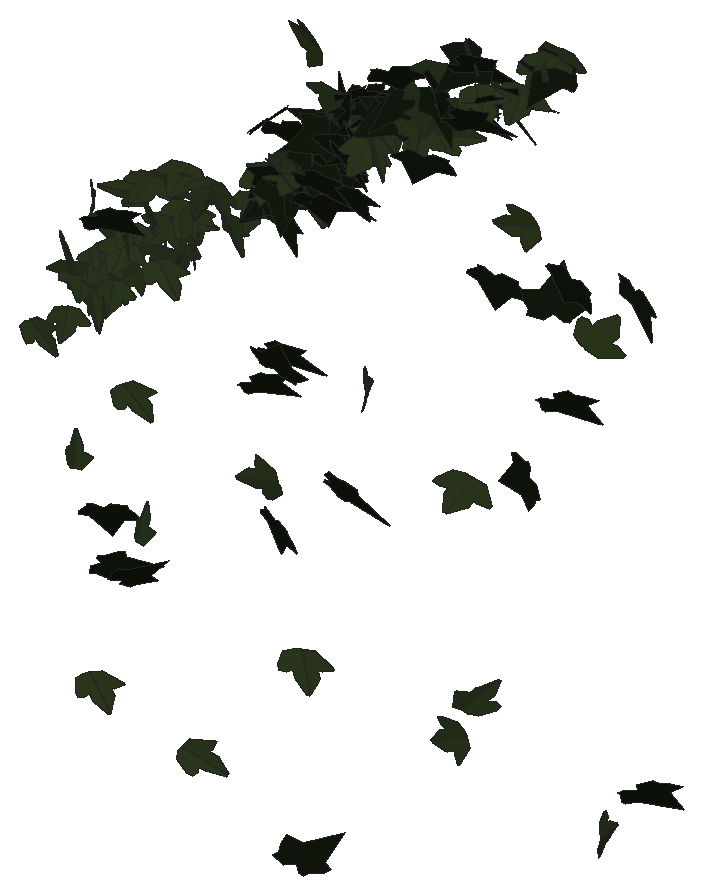
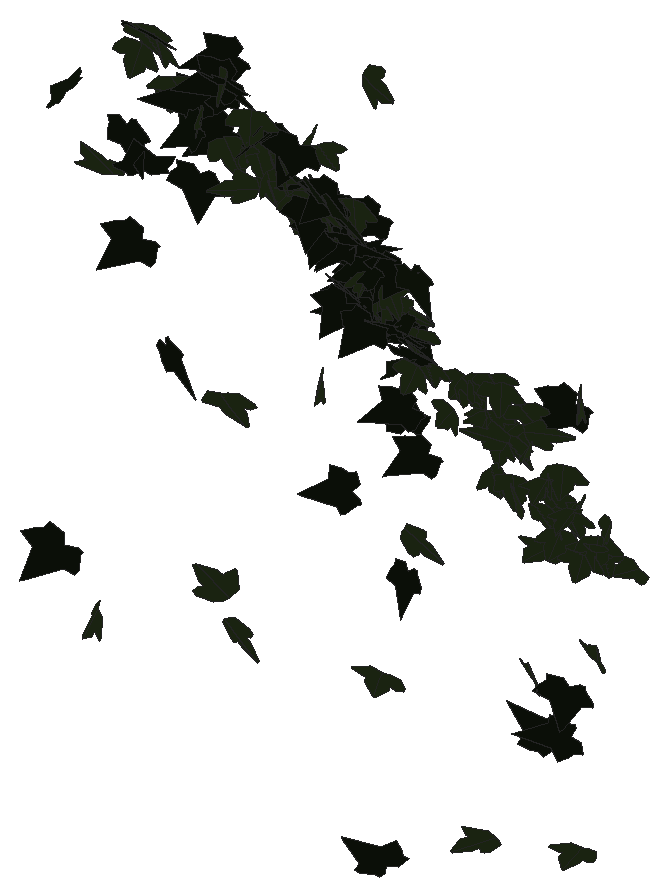
# SketchUp Ruby script. Lengths in inches.
U = 1.inch
M = Sketchup.active_model
def pt(a) = Geom::Point3d.new(a.map { |v| v * U })
def face(e, loops, mat)
  f = e.add_face(loops[0].map { |a| pt(a) })
  loops[1..].each { |l| e.add_face(l.map { |a| pt(a) }).erase! }
  f.material = f.back_material = mat if mat
  f
end
# faces: each face lists its corners as indices into pts; further lists are holes
def faces(e, pts, list, mat = nil) = list.each { |f| face(e, (f[0].is_a?(Array) ? f : [f]).map { |l| l.map { |i| pts[i] } }, mat) }
# xy, xz, yz: faces in a plane at the given z, y or x. An outline is a flat list of corners, or four numbers for a rectangle; further outlines are holes
def ring(l) = l.size == 4 ? [[l[0], l[1]], [l[2], l[1]], [l[2], l[3]], [l[0], l[3]]] : l.each_slice(2).to_a
def flat(e, list, mat, &to3) = list.each { |f| face(e, (f[0].is_a?(Array) ? f : [f]).map { |l| ring(l).map { |u, v| to3.(u, v) } }, mat) }
def xy(e, z, list, mat = nil) = flat(e, list, mat) { |x, y| [x, y, z] }
def xz(e, y, list, mat = nil) = flat(e, list, mat) { |x, z| [x, y, z] }
def yz(e, x, list, mat = nil) = flat(e, list, mat) { |y, z| [x, y, z] }
def lines(e, pts, list) = list.each { |a, b| e.add_line(pt(pts[a]), pt(pts[b])) }
# prism: a flat outline (further loops are holes) pulled along v
def prism(e, loops, v, mat = nil)
  f = face(e, loops, mat); d = Geom::Vector3d.new(v.map { |x| x * U })
  f.pushpull(f.normal.samedirection?(d) ? d.length : -d.length)
end
def box(e, o, s, mat = nil) = prism(e, [[o, [o[0] + s[0], o[1], o[2]], [o[0] + s[0], o[1] + s[1], o[2]], [o[0], o[1] + s[1], o[2]]]], [0, 0, s[2]], mat)
def at(x, y, z, deg = 0) = Geom::Transformation.translation(pt([x, y, z])) * Geom::Transformation.rotation(ORIGIN, Z_AXIS, deg.degrees)
def axes(o, x, y, z) = Geom::Transformation.new([*x, 0, *y, 0, *z, 0, *pt(o).to_a, 1])
def part(name) = M.definitions.add(name)
# library, detail: a bought-in or finely detailed component or shape, given as its bounding box
def library(name, o, s) = part(name).tap { |d| box(d.entities, o, s) }
def detail(e, o, s) = box(e.add_group.entities, o, s)
def put(e, d, t, mat = nil) = e.add_instance(d, t).tap { |i| i.material = mat if mat }
def group(e, t, mat = nil) = e.add_group.tap { |g| g.transformation = t; g.material = mat if mat }.entities
root = M.entities
M.materials.add("1026 AP 7946 SUNNY SIDE UP").color = [254, 231, 186]
M.materials.add("efeu1").color = [18, 25, 13]
M.materials.add("efeu2").color = [43, 57, 29]
c1 = part("ivyleaf_10")
p = [[0,0.5,-0.03],[-0.0625,2.02,-0.43],[-0.19,2.01,-0.46],[-0.54,1.05,-0.29],[-0.52,0.625,-0.18],[-0.83,0.76,-0.28],
  [-1.16,0.64,-0.33],[-1.15,0.33,-0.24],[-0.77,-0.39,0.02],[-0.3,-0.51,0.16],[0.04,-0.48,0.23],[-0.02,2.01,-0.4375],
  [-0.06,2.01,-0.43],[0.04,-0.49,0.23],[0.67,-0.49,0.14],[1.38,0.36,-0.2],[1.375,0.51,-0.24],[0.81,0.65,-0.19],
  [0.62,0.59,-0.15],[0.6,1.09,-0.28],[0.5,1.23,-0.31]]
faces(c1.entities,p,[[0,1,2,3,4,5,6,7,8,9,10],[11,12,0,13,14,15,16,17,18,19,20]],"efeu2")
c2 = part("ivyleaf_9")
p = [[1.54,2.16,1.25],[1.36,2.04,1.19],[-0.21,0.99,0.68],[-0.71,1.11,0.82],[-0.85,0.86,0.67],[-0.8,0.17,0.21],
  [-0.9,-0.01,0.1],[-0.67,-0.16,-0.02],[-0.08,-0.08,-0.05],[-0.03,-0.6,-0.4],[0.65,-0.88,-0.66],[0.83,-0.6,-0.49],
  [1.29,-0.42,-0.43],[1.8125,-0.07,-0.26],[1.21,0.44,0.15]]
faces(c2.entities,p,[[0,1,2,3,4,5,6,7,8,9,10,11,12,13,14]],"efeu1")
put(root,c1,axes([109.65,214.06,261.58],[-0.19808,0.18062,-0.01715],[-0.00079,-0.02186,-0.2266],[-0.28536,-0.12531,0.01253]),"1026 AP 7946 SUNNY SIDE UP")
put(root,c1,axes([109.84,214.1,261.2],[-0.29659,-0.12864,-0.00987],[0.02997,-0.01231,-0.23429],[0.20053,-0.18843,0.02042]),"1026 AP 7946 SUNNY SIDE UP")
put(root,c1,axes([109.68,213.29,260.41],[0.22874,0.0138,0.16664],[0.25222,0.0206,-0.15037],[-0.03858,0.21651,0.00497]),"1026 AP 7946 SUNNY SIDE UP")
put(root,c1,axes([109.94,214.14,261.09],[0.31539,0.08814,-0.00082],[0.00227,-0.0065,-0.22564],[-0.13859,0.20047,-0.00555]),"1026 AP 7946 SUNNY SIDE UP")
put(root,c1,axes([110.07,213.61,260.64],[0.20831,0.16899,-0.05013],[-0.04684,-0.03969,-0.22144],[-0.27294,0.13578,-0.00026]),"1026 AP 7946 SUNNY SIDE UP")
put(root,c1,axes([110.12,214.17,260.87],[-0.35185,-0.02632,-0.02014],[0.03536,-0.02645,-0.23036],[0.03733,-0.22304,0.02835]),"1026 AP 7946 SUNNY SIDE UP")
put(root,c1,axes([110.41,214.09,261.53],[0.35954,-0.00397,-0.0298],[-0.04586,-0.02417,-0.23438],[0.00139,0.22921,-0.02387]),"1026 AP 7946 SUNNY SIDE UP")
put(root,c1,axes([110.34,214.17,261.63],[0.096,0.2101,0.07603],[0.04559,0.06713,-0.22482],[-0.34654,0.06703,-0.00852]),"1026 AP 7946 SUNNY SIDE UP")
put(root,c1,axes([110.56,213.22,258.35],[0.29275,-0.09652,0.09081],[-0.10831,0.05904,0.21549],[-0.17536,-0.19759,0.0185]),"1026 AP 7946 SUNNY SIDE UP")
put(root,c1,axes([110.56,214.12,262.31],[-0.29961,-0.12774,-0.00939],[0.02754,-0.01111,-0.23558],[0.1994,-0.1904,0.01843]),"1026 AP 7946 SUNNY SIDE UP")
put(root,c1,axes([110.53,214.26,261.17],[-0.26411,-0.14621,-0.05641],[0.11074,-0.00049,-0.22462],[0.21859,-0.17641,0.04564]),"1026 AP 7946 SUNNY SIDE UP")
put(root,c1,axes([110.75,214.16,261.83],[0.32097,0.07208,-0.05912],[-0.07057,-0.04516,-0.22158],[-0.12698,0.20729,-0.0263]),"1026 AP 7946 SUNNY SIDE UP")
put(root,c1,axes([111.0625,214.2,262.9],[0.00692,0.04698,0.23371],[-0.25893,-0.1586,0.03624],[0.25566,-0.1619,0.03038]),"1026 AP 7946 SUNNY SIDE UP")
put(root,c1,axes([110.97,214.18,261.47],[0.27133,-0.074,-0.13753],[-0.18288,0.06576,-0.19265],[0.15453,0.20775,0.01348]),"1026 AP 7946 SUNNY SIDE UP")
put(root,c1,axes([110.95,213.14,263.14],[0.01472,-0.07788,-0.26817],[-0.07341,0.25568,-0.07917],[0.42021,0.04739,-0.00444]),"1026 AP 7946 SUNNY SIDE UP")
put(root,c1,axes([110.76,214.22,262.14],[0.14334,-0.18782,0.08225],[0.15104,-0.03888,-0.2047],[0.28389,0.11552,0.06738]),"1026 AP 7946 SUNNY SIDE UP")
put(root,c1,axes([110.78,213.53,261.11],[0.25159,-0.14485,0.05846],[0.10204,-0.01312,-0.21986],[0.22284,0.16954,0.03466]),"1026 AP 7946 SUNNY SIDE UP")
put(root,c1,axes([110.82,213.35,261.27],[-0.00209,0.21932,-0.04218],[0.00118,-0.04219,-0.22619],[-0.35117,-0.00145,-0.00051]),"1026 AP 7946 SUNNY SIDE UP")
put(root,c1,axes([110.8125,214.28,262.07],[0.17056,0.18859,0.05827],[0.04538,0.04741,-0.22384],[-0.30576,0.11224,-0.00072]),"1026 AP 7946 SUNNY SIDE UP")
put(root,c1,axes([110.91,213.72,261.36],[0.17244,0.1867,-0.06058],[-0.05157,-0.05016,-0.22334],[-0.30395,0.11443,0.00352]),"1026 AP 7946 SUNNY SIDE UP")
put(root,c2,axes([111.1,213.28,257.64],[0.25455,0.16438,-0.07515],[-0.06221,-0.06447,-0.23747],[-0.27647,0.16586,-0.01576]),"1026 AP 7946 SUNNY SIDE UP")
put(root,c1,axes([110.97,213.16,254.55],[0.25745,0.15708,0.08997],[0.11874,0.04575,-0.23274],[-0.25569,0.1794,-0.0175]),"1026 AP 7946 SUNNY SIDE UP")
put(root,c1,axes([111.22,214.2,262.69],[-0.20711,0.18199,-0.03084],[0.0151,-0.03124,-0.23137],[-0.28988,-0.13165,0.00998]),"1026 AP 7946 SUNNY SIDE UP")
put(root,c1,axes([111.33,214.15,263.24],[0.28997,0.09164,-0.108],[-0.15605,-0.03677,-0.21211],[-0.15446,0.20918,0.01153]),"1026 AP 7946 SUNNY SIDE UP")
put(root,c2,axes([111.12,213.13,262.96],[0.3176,0.15922,0.09298],[0.13086,0.03831,-0.26391],[-0.25552,0.21751,-0.01959]),"1026 AP 7946 SUNNY SIDE UP")
put(root,c1,axes([111.28,214.36,261.52],[0.21264,-0.18195,0.04398],[-0.02947,0.0405,0.2336],[-0.29276,-0.13623,0.00843]),"1026 AP 7946 SUNNY SIDE UP")
put(root,c2,axes([111.14,213.23,256.7],[0.07663,0.12792,-0.2056],[0.10106,0.18975,0.14206],[0.35978,-0.08055,0.00389]),"1026 AP 7946 SUNNY SIDE UP")
put(root,c1,axes([111.44,214.35,261.91],[-0.35273,-0.05295,0.03841],[-0.04765,-0.03419,-0.23614],[0.09031,-0.22487,0.02544]),"1026 AP 7946 SUNNY SIDE UP")
put(root,c1,axes([111.64,214.16,262.54],[0.31646,-0.06795,-0.10537],[-0.16239,0.01119,-0.21777],[0.10351,0.2253,-0.01952]),"1026 AP 7946 SUNNY SIDE UP")
put(root,c2,axes([111.52,213.26,256.54],[0.24366,0.18769,-0.02528],[0.00706,0.02943,0.25042],[0.29777,-0.15428,0.01475]),"1026 AP 7946 SUNNY SIDE UP")
put(root,c1,axes([111.78,214.27,262.51],[-0.33307,0.08327,-0.00535],[-0.02113,-0.04927,-0.22886],[-0.12952,-0.20609,0.05108]),"1026 AP 7946 SUNNY SIDE UP")
put(root,c1,axes([111.8125,214.43,261.99],[0.03711,0.22603,-0.0537],[-0.13522,-0.04136,-0.21974],[-0.33925,0.04121,0.08171]),"1026 AP 7946 SUNNY SIDE UP")
put(root,c1,axes([111.83,214.1875,263.47],[-0.36502,-0.03533,0.01577],[-0.01924,-0.02229,-0.24114],[0.05753,-0.23159,0.01941]),"1026 AP 7946 SUNNY SIDE UP")
put(root,c1,axes([111.875,213.22,257.48],[0.27607,-0.15306,0.08127],[-0.07448,0.06667,0.23962],[-0.26097,-0.18095,0.01759]),"1026 AP 7946 SUNNY SIDE UP")
put(root,c1,axes([111.6875,213.13,260.02],[0.25173,0.08709,0.14865],[0.20323,0.06323,-0.18731],[-0.16905,0.2057,-0.00382]),"1026 AP 7946 SUNNY SIDE UP")
put(root,c1,axes([111.97,214.1875,263.63],[0.32235,0.08199,-0.07445],[-0.09773,-0.04009,-0.22727],[-0.14194,0.2138,-0.01259]),"1026 AP 7946 SUNNY SIDE UP")
put(root,c1,axes([111.74,214.32,262.6],[-0.04798,0.01248,0.23287],[0.30099,0.12306,0.02034],[-0.18984,0.19196,-0.0266]),"1026 AP 7946 SUNNY SIDE UP")
put(root,c1,axes([112.01,214.21,262.9375],[0.3458,0.08689,-0.02806],[-0.02796,-0.03015,-0.24278],[-0.14066,0.2196,-0.02072]),"1026 AP 7946 SUNNY SIDE UP")
put(root,c1,axes([112.11,214.2,262.875],[0.10937,0.21723,0.03423],[0.00698,0.03217,-0.23473],[-0.34519,0.06948,0.0061]),"1026 AP 7946 SUNNY SIDE UP")
put(root,c1,axes([112.16,213.36,262.3],[0.28171,0.10065,0.10538],[0.15484,0.03155,-0.21065],[-0.16325,0.20359,-0.01795]),"1026 AP 7946 SUNNY SIDE UP")
put(root,c1,axes([112.39,214.27,263.32],[-0.09104,-0.20297,0.09645],[-0.0037,-0.09733,-0.21679],[0.35221,-0.05349,0.02265]),"1026 AP 7946 SUNNY SIDE UP")
put(root,c1,axes([112.4,214.32,263.43],[-0.1412,-0.17519,0.14198],[-0.01035,-0.14745,-0.19697],[0.3513,-0.07476,0.05126]),"1026 AP 7946 SUNNY SIDE UP")
put(root,c1,axes([112.54,214.29,263.41],[-0.30681,0.08481,-0.09525],[0.10579,-0.07459,-0.21607],[-0.16717,-0.20284,0.03807]),"1026 AP 7946 SUNNY SIDE UP")
put(root,c1,axes([112.84,213.37,262.82],[-0.02303,0.08372,0.22337],[-0.24115,0.15916,-0.07321],[-0.27369,-0.14728,0.04571]),"1026 AP 7946 SUNNY SIDE UP")
put(root,c1,axes([112.7,214.46,262.84],[-0.27844,0.11345,-0.11503],[0.10488,-0.0998,-0.2128],[-0.22805,-0.18442,0.04259]),"1026 AP 7946 SUNNY SIDE UP")
put(root,c1,axes([113.01,213.07,254.01],[0.11744,0.12839,0.21009],[0.20339,0.15788,-0.15082],[-0.31856,0.14813,-0.01885]),"1026 AP 7946 SUNNY SIDE UP")
put(root,c1,axes([113.26,214.29,263.48],[0.37004,-0.04836,0.03153],[0.03891,-0.03209,-0.24621],[0.08139,0.23517,-0.02565]),"1026 AP 7946 SUNNY SIDE UP")
put(root,c1,axes([113.32,214.63,263.48],[-0.34034,0.09639,-0.04763],[0.05173,-0.04057,-0.24316],[-0.16033,-0.2177,0.02266]),"1026 AP 7946 SUNNY SIDE UP")
put(root,c2,axes([113.6,214.3,265.11],[-0.07499,0.234,-0.04059],[0.00641,-0.04073,-0.24622],[-0.37342,-0.04769,0.00392]),"1026 AP 7946 SUNNY SIDE UP")
put(root,c2,axes([113.67,214.46,263.68],[-0.38039,-0.02921,-0.00401],[0.01018,-0.02272,-0.25001],[0.04517,-0.24087,0.02262]),"1026 AP 7946 SUNNY SIDE UP")
put(root,c1,axes([113.5,214.27,264],[0.34435,0.08581,0.02282],[0.04045,-0.0064,-0.24184],[-0.13316,0.21997,-0.01446]),"1026 AP 7946 SUNNY SIDE UP")
put(root,c2,axes([113.85,214.24,264.17],[0.11422,0.11143,-0.21305],[-0.19474,-0.16655,-0.13782],[-0.31491,0.14341,0.00796]),"1026 AP 7946 SUNNY SIDE UP")
put(root,c1,axes([114.02,214.23,264.27],[0.08626,-0.036,-0.24547],[-0.37467,0.02697,-0.06061],[0.05441,0.24282,-0.02819]),"1026 AP 7946 SUNNY SIDE UP")
put(root,c2,axes([113.93,214.3125,263.85],[-0.38288,0.00832,0.0003],[-0.00141,-0.01905,-0.25034],[-0.01302,-0.24276,0.01822]),"1026 AP 7946 SUNNY SIDE UP")
put(root,c2,axes([113.7,214.45,263.35],[0.04602,-0.22501,0.0856],[0.0695,-0.0785,-0.23194],[0.37141,0.04257,0.0328]),"1026 AP 7946 SUNNY SIDE UP")
put(root,c2,axes([114.18,214.55,263.99],[-0.29132,0.05734,0.1546],[-0.24974,-0.03424,-0.18914],[-0.03458,-0.23575,0.06358]),"1026 AP 7946 SUNNY SIDE UP")
put(root,c2,axes([113.83,214.33,263.89],[-0.09397,-0.23701,0.00604],[0.01106,-0.0092,-0.25169],[0.37269,-0.05948,0.00899]),"1026 AP 7946 SUNNY SIDE UP")
put(root,c2,axes([113.75,214.26,264.25],[0.34151,-0.10988,-0.03709],[-0.05939,0.0036,-0.25033],[0.17153,0.22002,-0.01282]),"1026 AP 7946 SUNNY SIDE UP")
put(root,c1,axes([114.01,214.39,264.66],[-0.06473,-0.23961,0.04875],[-0.00325,-0.04902,-0.25066],[0.38444,-0.04076,0.00609]),"1026 AP 7946 SUNNY SIDE UP")
put(root,c2,axes([113.87,214.27,265.07],[0.33813,0.1157,-0.01553],[-0.00635,-0.02559,-0.25082],[-0.1835,0.21409,-0.01995]),"1026 AP 7946 SUNNY SIDE UP")
put(root,c1,axes([114.46,213.24,259.34],[-0.14457,0.04296,0.24509],[-0.37975,-0.01529,-0.0935],[-0.00159,-0.25437,0.04547]),"1026 AP 7946 SUNNY SIDE UP")
put(root,c2,axes([114.16,214.72,264.12],[0.30045,0.15061,0.03115],[0.04175,0.01376,-0.2505],[-0.23764,0.19283,-0.00463]),"1026 AP 7946 SUNNY SIDE UP")
put(root,c1,axes([114.375,214.3125,264.22],[-0.3463,0.08386,0.07204],[-0.11845,-0.0042,-0.24089],[-0.12362,-0.23089,0.02902]),"1026 AP 7946 SUNNY SIDE UP")
put(root,c2,axes([114.15,213.24,261.01],[0.27576,0.13259,0.10914],[0.1471,0.05029,-0.22569],[-0.22178,0.19822,-0.01399]),"1026 AP 7946 SUNNY SIDE UP")
put(root,c1,axes([114.33,214.55,263.89],[0.33701,0.10392,0.05783],[0.09477,0.00239,-0.24417],[-0.15921,0.22139,-0.02293]),"1026 AP 7946 SUNNY SIDE UP")
put(root,c2,axes([114.54,213.26,258.61],[0.29154,-0.03541,-0.18252],[-0.27954,0.00786,-0.19346],[0.04887,0.25619,-0.01777]),"1026 AP 7946 SUNNY SIDE UP")
put(root,c1,axes([114.54,214.41,264.79],[0.04496,0.23805,0.00179],[-0.0171,0.0017,-0.24673],[-0.37393,0.02855,0.0115]),"1026 AP 7946 SUNNY SIDE UP")
put(root,c2,axes([114.73,214.35,265.14],[-0.21557,-0.11089,0.18364],[-0.19402,-0.13061,-0.18159],[0.2681,-0.18368,0.01625]),"1026 AP 7946 SUNNY SIDE UP")
put(root,c2,axes([114.36,214.41,265.01],[0.36802,-0.07952,0.03668],[0.05035,-0.01778,-0.25467],[0.12772,0.23614,-0.00528]),"1026 AP 7946 SUNNY SIDE UP")
put(root,c2,axes([114.95,214.47,265.28],[-0.19106,0.08458,0.19848],[-0.30043,0.04756,-0.14573],[-0.13694,-0.22235,0.04278]),"1026 AP 7946 SUNNY SIDE UP")
put(root,c2,axes([114.59,214.29,264.74],[-0.13231,-0.23205,0.03915],[0.0133,-0.04471,-0.25345],[0.36983,-0.08141,0.02312]),"1026 AP 7946 SUNNY SIDE UP")
put(root,c2,axes([114.57,213.23,261.42],[0.36333,-0.06749,0.04934],[-0.05594,0.04849,0.24551],[-0.11788,-0.23102,0.03559]),"1026 AP 7946 SUNNY SIDE UP")
put(root,c2,axes([114.6,214.54,264.39],[0.37143,0.05999,-0.04622],[-0.06198,-0.028,-0.25062],[-0.10054,0.23887,-0.01626]),"1026 AP 7946 SUNNY SIDE UP")
put(root,c2,axes([114.67,214.74,264.35],[0.21223,0.1964,0.06584],[0.06935,0.04581,-0.24502],[-0.31672,0.14164,-0.00953]),"1026 AP 7946 SUNNY SIDE UP")
put(root,c1,axes([114.83,214.35,265.95],[-0.38225,0.00037,0.05294],[-0.08054,-0.02153,-0.24962],[0.00643,-0.24754,0.02034]),"1026 AP 7946 SUNNY SIDE UP")
put(root,c2,axes([114.95,214.6,264.58],[-0.36717,0.08381,-0.01157],[0.00675,-0.02259,-0.2549],[-0.13289,-0.23271,0.01902]),"1026 AP 7946 SUNNY SIDE UP")
put(root,c2,axes([114.54,213.2,261.74],[0.34512,0.04874,0.10037],[0.15471,0.00392,-0.231],[-0.07261,0.23999,-0.01515]),"1026 AP 7946 SUNNY SIDE UP")
put(root,c2,axes([114.54,214.39,264.14],[0.33946,-0.0529,0.10845],[0.16348,-0.01913,-0.22903],[0.08802,0.23955,0.00713]),"1026 AP 7946 SUNNY SIDE UP")
put(root,c2,axes([115.13,214.3,265.15],[0.09393,0.09882,-0.23024],[-0.18137,-0.19208,-0.12008],[-0.33965,0.1299,0.00045]),"1026 AP 7946 SUNNY SIDE UP")
put(root,c2,axes([115.17,214.38,265.93],[-0.20462,0.20659,-0.00038],[-0.02575,-0.01212,-0.25073],[-0.32383,-0.12958,0.02017]),"1026 AP 7946 SUNNY SIDE UP")
put(root,c2,axes([114.98,213.73,264.39],[0.29089,0.13982,-0.07077],[-0.07097,-0.05525,-0.23864],[-0.23502,0.18974,-0.01553]),"1026 AP 7946 SUNNY SIDE UP")
put(root,c2,axes([115.17,214.1875,265.73],[0.0151,0.01439,0.25765],[-0.0295,0.24954,-0.01259],[-0.39267,-0.01819,0.01085]),"1026 AP 7946 SUNNY SIDE UP")
put(root,c2,axes([114.92,214.45,265.33],[0.36725,-0.04072,-0.05432],[-0.0859,-0.00849,-0.24364],[0.05947,0.23924,-0.01645]),"1026 AP 7946 SUNNY SIDE UP")
put(root,c1,axes([115.46,213.07,267.57],[0.03235,0.02424,-0.30233],[-0.30195,0.22431,0.00653],[0.35131,0.19056,0.03345]),"1026 AP 7946 SUNNY SIDE UP")
put(root,c1,axes([115.35,214.3,265.41],[0.13917,-0.21307,-0.1083],[-0.06428,0.09554,-0.23713],[0.36717,0.09749,-0.00047]),"1026 AP 7946 SUNNY SIDE UP")
put(root,c1,axes([115.14,213.18,256.41],[0.37991,0.07493,0.07284],[0.11635,-0.00235,-0.25951],[-0.11205,0.25162,-0.02251]),"1026 AP 7946 SUNNY SIDE UP")
put(root,c2,axes([115.2,214.34,266.0625],[0.30008,0.14255,0.05828],[0.07069,0.03299,-0.2452],[-0.23007,0.19607,0.00067]),"1026 AP 7946 SUNNY SIDE UP")
put(root,c2,axes([115.16,213.08,252.79],[-0.09523,-0.00785,0.26181],[0.38594,0.06655,0.06276],[-0.1046,0.25268,-0.00681]),"1026 AP 7946 SUNNY SIDE UP")
put(root,c2,axes([115.3,214.43,265.43],[0.28746,0.15549,-0.04285],[-0.03298,-0.04073,-0.24685],[-0.2513,0.18321,-0.01662]),"1026 AP 7946 SUNNY SIDE UP")
put(root,c2,axes([115.26,214.04,265.18],[0.35428,-0.05007,-0.08324],[-0.1324,-0.01022,-0.23624],[0.06855,0.23905,-0.02608]),"1026 AP 7946 SUNNY SIDE UP")
put(root,c1,axes([115.46,214.4,265.42],[-0.34887,0.09665,0.02727],[-0.08397,-0.06105,-0.23677],[-0.13306,-0.21488,0.07792]),"1026 AP 7946 SUNNY SIDE UP")
put(root,c2,axes([115.64,214.38,266.12],[-0.26583,0.17469,-0.03125],[0.01472,-0.03442,-0.25002],[-0.27868,-0.16845,0.01659]),"1026 AP 7946 SUNNY SIDE UP")
put(root,c2,axes([115.27,213.18,265.12],[0.36828,0.05586,0.03152],[0.05187,-0.00808,-0.2476],[-0.08539,0.23603,-0.01447]),"1026 AP 7946 SUNNY SIDE UP")
put(root,c2,axes([115.58,214.46,265.69],[0.17479,0.21668,-0.02644],[-0.00886,-0.02733,-0.25092],[-0.3432,0.11106,-0.00699]),"1026 AP 7946 SUNNY SIDE UP")
put(root,c1,axes([115.53,214.37,265.61],[0.37841,-0.04665,-0.00115],[-0.0035,-0.00704,-0.25246],[0.07328,0.24055,-0.00615]),"1026 AP 7946 SUNNY SIDE UP")
put(root,c1,axes([115.72,214.375,265.78],[-0.37136,-0.0607,-0.03047],[0.0532,-0.01471,-0.25023],[0.0916,-0.23752,0.0218]),"1026 AP 7946 SUNNY SIDE UP")
put(root,c2,axes([115.625,213.61,264.81],[0.36053,0.07072,-0.04807],[-0.06542,-0.02462,-0.24707],[-0.11646,0.23276,-0.01002]),"1026 AP 7946 SUNNY SIDE UP")
put(root,c1,axes([115.8125,214.46,265.68],[-0.37936,-0.04168,-0.00822],[0.01699,-0.01723,-0.25159],[0.06445,-0.24077,0.01797]),"1026 AP 7946 SUNNY SIDE UP")
put(root,c2,axes([116.03,214.43,265.95],[-0.31682,-0.11021,0.09194],[-0.07844,-0.09118,-0.23093],[0.2094,-0.2009,0.0526]),"1026 AP 7946 SUNNY SIDE UP")
put(root,c2,axes([116.09,214.48,266.21],[-0.36104,-0.0093,-0.09334],[0.13737,-0.09157,-0.21905],[-0.04022,-0.22921,0.08974]),"1026 AP 7946 SUNNY SIDE UP")
put(root,c2,axes([115.95,214.39,266.71],[0.27478,0.17532,-0.01432],[0.00568,-0.02456,-0.25434],[-0.27661,0.17366,-0.01945]),"1026 AP 7946 SUNNY SIDE UP")
put(root,c1,axes([115.9,214.35,265.93],[0.36376,0.01752,0.1081],[0.16607,-0.00986,-0.23848],[-0.01866,0.25379,-0.01524]),"1026 AP 7946 SUNNY SIDE UP")
put(root,c2,axes([115.77,213.24,259.73],[0.35755,-0.0835,0.10841],[0.14383,-0.05654,-0.24905],[0.15549,0.2443,-0.01891]),"1026 AP 7946 SUNNY SIDE UP")
put(root,c1,axes([116.34,214.51,266.375],[0.23012,-0.16614,-0.11709],[-0.10426,0.09165,-0.22734],[0.29797,0.16038,0.01088]),"1026 AP 7946 SUNNY SIDE UP")
put(root,c1,axes([116.36,213.25,261.63],[0.0336,-0.07352,-0.2642],[-0.03709,0.25533,-0.07606],[0.41722,0.02862,0.01451]),"1026 AP 7946 SUNNY SIDE UP")
put(root,c1,axes([116.39,213.22,266.02],[0.28277,0.13859,-0.10073],[-0.11228,-0.06866,-0.23407],[-0.24269,0.19324,-0.00907]),"1026 AP 7946 SUNNY SIDE UP")
put(root,c1,axes([116.49,214.4,265.81],[0.39214,0.05005,-0.01038],[-0.0069,-0.03043,-0.26052],[-0.08006,0.24774,-0.02837]),"1026 AP 7946 SUNNY SIDE UP")
put(root,c1,axes([116.51,214.43,265.93],[-0.06487,-0.23925,0.08128],[0.09321,-0.08823,-0.24009],[0.38569,-0.01892,0.07169]),"1026 AP 7946 SUNNY SIDE UP")
put(root,c1,axes([116.66,213.15,266.14],[-0.05113,0.24225,-0.04258],[0.01634,-0.04169,-0.252],[-0.38644,-0.03381,-0.00502]),"1026 AP 7946 SUNNY SIDE UP")
put(root,c1,axes([116.82,214.41,266.33],[-0.21285,-0.21377,0.05108],[-0.01952,-0.05212,-0.26038],[0.34494,-0.13486,0.01678]),"1026 AP 7946 SUNNY SIDE UP")
put(root,c1,axes([116.84,214.54,267.03],[-0.35661,-0.10633,-0.00007],[0.01245,-0.01815,-0.25734],[0.16673,-0.22607,0.01907]),"1026 AP 7946 SUNNY SIDE UP")
put(root,c2,axes([116.81,214.48,266.51],[0.05925,-0.24594,-0.02416],[-0.0214,0.02021,-0.25599],[0.38768,0.0387,-0.01044]),"1026 AP 7946 SUNNY SIDE UP")
put(root,c2,axes([116.84,214.53,266.69],[0.01038,-0.17212,0.18596],[0.01155,-0.18133,-0.17851],[0.39312,0.00987,0.00034]),"1026 AP 7946 SUNNY SIDE UP")
put(root,c1,axes([116.81,214.66,265.75],[0.00071,0.01911,0.26225],[0.18007,0.22738,-0.01647],[-0.35856,0.11423,-0.00775]),"1026 AP 7946 SUNNY SIDE UP")
put(root,c1,axes([117.24,214.65,266.4],[-0.3124,-0.14093,0.09005],[-0.10056,-0.06209,-0.25096],[0.24132,-0.20832,0.012]),"1026 AP 7946 SUNNY SIDE UP")
put(root,c2,axes([117.39,213.4,266.11],[0.21395,0.1536,-0.14928],[-0.15647,-0.10658,-0.21199],[-0.29393,0.16854,0.00419]),"1026 AP 7946 SUNNY SIDE UP")
put(root,c1,axes([117.46,214.49,267.55],[-0.21486,0.21051,0.02896],[-0.04893,0.01179,-0.25769],[-0.3301,-0.13877,0.01934]),"1026 AP 7946 SUNNY SIDE UP")
put(root,c2,axes([117.61,214.5,267.46],[-0.41194,-0.02173,-0.02066],[0.03408,-0.02107,-0.26992],[0.03144,-0.26189,0.02188]),"1026 AP 7946 SUNNY SIDE UP")
put(root,c2,axes([117.36,214.44,266.52],[0.37938,0.07255,0.05967],[0.09809,-0.0088,-0.25825],[-0.10756,0.24787,-0.02506]),"1026 AP 7946 SUNNY SIDE UP")
put(root,c1,axes([117.78,214.71,266.82],[-0.16006,0.22563,0.08543],[-0.11003,0.05691,-0.25159],[-0.36089,-0.11742,0.03882]),"1026 AP 7946 SUNNY SIDE UP")
put(root,c2,axes([117.5,214.3,267.42],[0.33046,0.06922,0.14304],[0.22086,0.01282,-0.22618],[-0.10227,0.25134,-0.02627]),"1026 AP 7946 SUNNY SIDE UP")
put(root,c2,axes([117.72,214.88,266.68],[0.35239,-0.1303,-0.00643],[-0.03028,-0.02225,-0.26552],[0.20281,0.22307,-0.02848]),"1026 AP 7946 SUNNY SIDE UP")
put(root,c2,axes([117.93,214.03,267.01],[0.19806,0.22098,0.02292],[0.03118,0.01284,-0.26172],[-0.34763,0.12705,-0.01041]),"1026 AP 7946 SUNNY SIDE UP")
put(root,c1,axes([117.97,214.07,267.16],[0.247,0.19784,0.04074],[0.05269,0.0224,-0.25981],[-0.31249,0.16015,-0.01161]),"1026 AP 7946 SUNNY SIDE UP")
put(root,c1,axes([118.36,213.08,256.17],[0.23269,-0.12067,-0.20575],[-0.25124,0.11884,-0.19591],[0.26613,0.21769,-0.00506]),"1026 AP 7946 SUNNY SIDE UP")
put(root,c2,axes([117.93,214.49,266.94],[0.30313,0.00842,0.18075],[0.27297,0.03013,-0.19787],[-0.04162,0.25889,0.01868]),"1026 AP 7946 SUNNY SIDE UP")
put(root,c1,axes([118.34,213.3,260.62],[0.40576,0.04059,-0.09037],[-0.12964,-0.03934,-0.26814],[-0.07996,0.26977,-0.02386]),"1026 AP 7946 SUNNY SIDE UP")
put(root,c2,axes([118.1875,213.28,267.16],[0.3162,0.07006,0.14402],[0.21334,0.03375,-0.2189],[-0.12111,0.24235,-0.00959]),"1026 AP 7946 SUNNY SIDE UP")
put(root,c1,axes([118.4375,214.54,267.15],[0.34107,0.13558,-0.06025],[-0.08538,-0.02487,-0.26355],[-0.21642,0.22348,0.00903]),"1026 AP 7946 SUNNY SIDE UP")
put(root,c1,axes([118.59,213.11,256.8125],[-0.16614,-0.2056,0.15618],[0.08741,0.14291,0.23859],[-0.39317,0.11865,-0.01295]),"1026 AP 7946 SUNNY SIDE UP")
put(root,c1,axes([118.74,214.54,267.75],[0.33602,-0.13257,0.08747],[0.10255,-0.05713,-0.25904],[0.22599,0.22303,-0.01251]),"1026 AP 7946 SUNNY SIDE UP")
put(root,c1,axes([118.875,214.99,267.8],[-0.40405,0.05905,-0.02758],[0.03074,-0.0352,-0.27009],[-0.09744,-0.25598,0.02917]),"1026 AP 7946 SUNNY SIDE UP")
put(root,c2,axes([118.97,213.23,264.6],[0.31956,0.07249,-0.15568],[-0.20385,-0.08355,-0.22079],[-0.16795,0.23934,-0.02823]),"1026 AP 7946 SUNNY SIDE UP")
put(root,c1,axes([119.125,214.52,267.89],[0.39202,-0.02257,-0.09191],[-0.14276,-0.02056,-0.25651],[0.0224,0.26395,-0.02628]),"1026 AP 7946 SUNNY SIDE UP")
put(root,c2,axes([119.18,214.55,267.88],[-0.38741,-0.06551,-0.07773],[0.13517,-0.0385,-0.25624],[0.07922,-0.25467,0.05711]),"1026 AP 7946 SUNNY SIDE UP")
put(root,c2,axes([119.5625,213.32,261.15],[0.04212,-0.0109,-0.28795],[-0.43951,0.00811,-0.02788],[0.01434,0.28061,-0.00874]),"1026 AP 7946 SUNNY SIDE UP")
put(root,c1,axes([119.74,213.11,265.83],[0.16561,-0.0677,-0.24252],[-0.33722,0.09747,-0.12736],[0.18491,0.23839,-0.01506]),"1026 AP 7946 SUNNY SIDE UP")
put(root,c2,axes([120.12,213.29,264.36],[-0.29535,-0.07299,0.18277],[0.26614,0.05506,0.20778],[-0.14328,0.25273,0.0092]),"1026 AP 7946 SUNNY SIDE UP")
put(root,c2,axes([120.46,213.28,265.04],[0.22407,0.00659,-0.23632],[-0.35263,-0.05353,-0.14539],[-0.07688,0.26473,-0.02191]),"1026 AP 7946 SUNNY SIDE UP")
put(root,c2,axes([120.3,213.14,262.89],[0.34882,0.13821,0.0651],[0.10147,0.01405,-0.26826],[-0.21579,0.23002,-0.0209]),"1026 AP 7946 SUNNY SIDE UP")
put(root,c1,axes([120.9,213.28,264.09],[0.37894,-0.01257,-0.12735],[0.19426,0.05166,0.24315],[0.01983,-0.26585,0.05165]),"1026 AP 7946 SUNNY SIDE UP")
put(root,c1,axes([121.24,213.1,255.4],[0.005,-0.06835,-0.28851],[0.02103,0.27942,-0.06856],[0.4522,-0.01224,0.00638]),"1026 AP 7946 SUNNY SIDE UP")
put(root,c2,axes([121.76,213.29,265.26],[0.09004,-0.24547,0.11212],[0.03626,-0.10781,-0.2603],[0.42156,0.0617,-0.00156]),"1026 AP 7946 SUNNY SIDE UP")
put(root,c2,axes([121.98,213.11,256.46],[0.31864,0.19132,0.08719],[0.1162,0.04316,-0.28622],[-0.30702,0.2149,-0.01784]),"1026 AP 7946 SUNNY SIDE UP")
